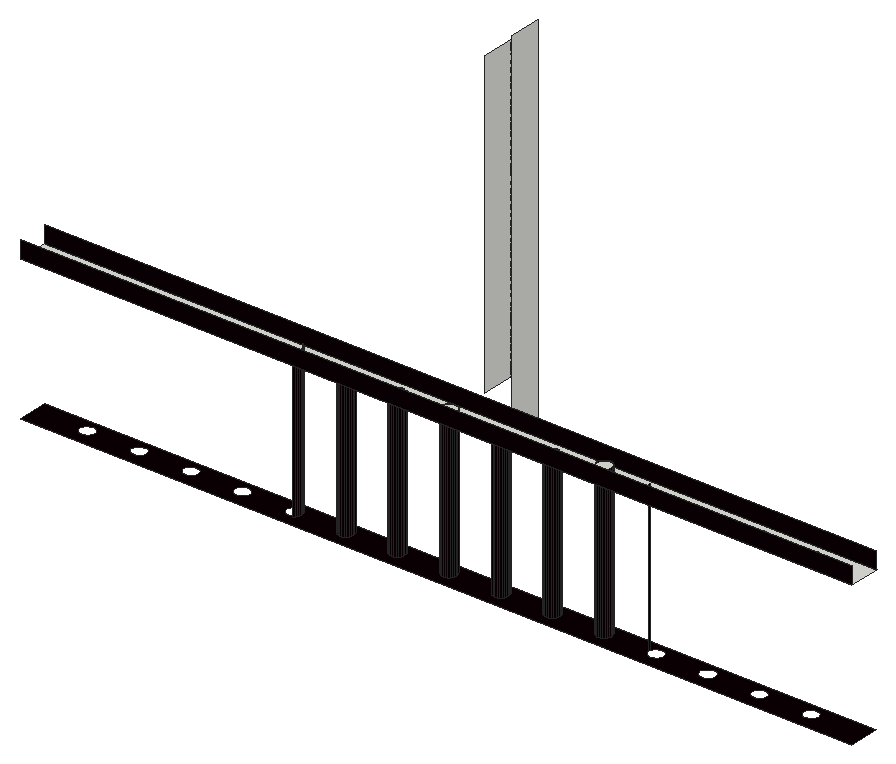
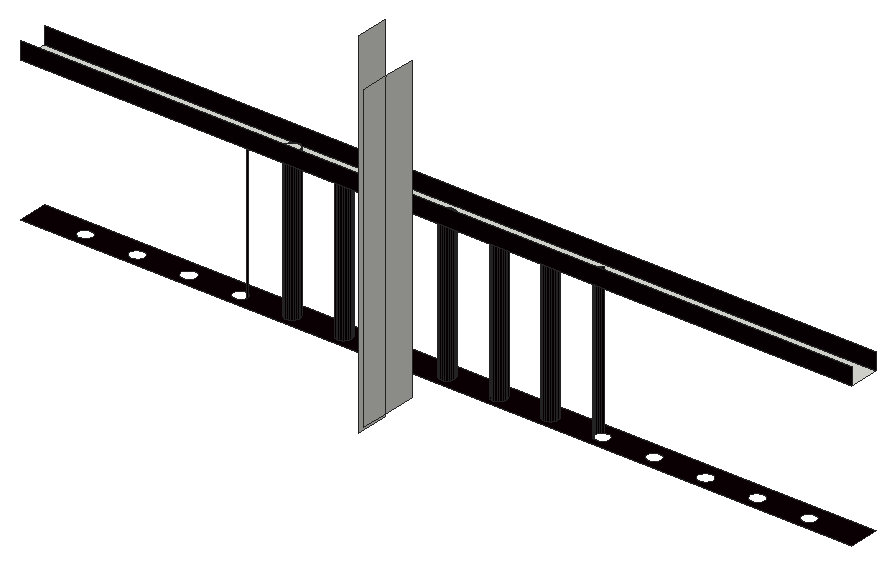
# SketchUp Ruby script. Lengths in inches.
U = 1.inch
M = Sketchup.active_model
def pt(a) = Geom::Point3d.new(a.map { |v| v * U })
def face(e, loops, mat)
  f = e.add_face(loops[0].map { |a| pt(a) })
  loops[1..].each { |l| e.add_face(l.map { |a| pt(a) }).erase! }
  f.material = f.back_material = mat if mat
  f
end
# faces: each face lists its corners as indices into pts; further lists are holes
def faces(e, pts, list, mat = nil) = list.each { |f| face(e, (f[0].is_a?(Array) ? f : [f]).map { |l| l.map { |i| pts[i] } }, mat) }
# xy, xz, yz: faces in a plane at the given z, y or x. An outline is a flat list of corners, or four numbers for a rectangle; further outlines are holes
def ring(l) = l.size == 4 ? [[l[0], l[1]], [l[2], l[1]], [l[2], l[3]], [l[0], l[3]]] : l.each_slice(2).to_a
def flat(e, list, mat, &to3) = list.each { |f| face(e, (f[0].is_a?(Array) ? f : [f]).map { |l| ring(l).map { |u, v| to3.(u, v) } }, mat) }
def xy(e, z, list, mat = nil) = flat(e, list, mat) { |x, y| [x, y, z] }
def xz(e, y, list, mat = nil) = flat(e, list, mat) { |x, z| [x, y, z] }
def yz(e, x, list, mat = nil) = flat(e, list, mat) { |y, z| [x, y, z] }
def lines(e, pts, list) = list.each { |a, b| e.add_line(pt(pts[a]), pt(pts[b])) }
# prism: a flat outline (further loops are holes) pulled along v
def prism(e, loops, v, mat = nil)
  f = face(e, loops, mat); d = Geom::Vector3d.new(v.map { |x| x * U })
  f.pushpull(f.normal.samedirection?(d) ? d.length : -d.length)
end
def box(e, o, s, mat = nil) = prism(e, [[o, [o[0] + s[0], o[1], o[2]], [o[0] + s[0], o[1] + s[1], o[2]], [o[0], o[1] + s[1], o[2]]]], [0, 0, s[2]], mat)
def at(x, y, z, deg = 0) = Geom::Transformation.translation(pt([x, y, z])) * Geom::Transformation.rotation(ORIGIN, Z_AXIS, deg.degrees)
def axes(o, x, y, z) = Geom::Transformation.new([*x, 0, *y, 0, *z, 0, *pt(o).to_a, 1])
def part(name) = M.definitions.add(name)
# library, detail: a bought-in or finely detailed component or shape, given as its bounding box
def library(name, o, s) = part(name).tap { |d| box(d.entities, o, s) }
def detail(e, o, s) = box(e.add_group.entities, o, s)
def put(e, d, t, mat = nil) = e.add_instance(d, t).tap { |i| i.material = mat if mat }
def group(e, t, mat = nil) = e.add_group.tap { |g| g.transformation = t; g.material = mat if mat }.entities
root = M.entities
M.materials.add("[Metal Seamed]").color = [11, 0, 4]
xy(root,156,[[439.47,72.62,439.03,72.67,438.62,72.83,438.26,73.09,437.99,73.43,437.8125,73.83,437.75,74.27,437.79,74.71,437.95,75.12,438.21,75.47,438.56,75.75,438.96,75.93,439.4,75.99,439.83,75.94,440.25,75.78,440.6,75.52,440.875,75.18,441.05,74.78,441.12,74.34,441.07,73.9,440.91,73.49,440.65,73.14,440.31,72.86,439.9,72.68],[451.09,72.62,450.66,72.67,450.25,72.83,449.89,73.09,449.61,73.43,449.4375,73.83,449.37,74.27,449.42,74.71,449.58,75.12,449.84,75.47,450.18,75.75,450.59,75.93,451.02,75.99,451.46,75.94,451.87,75.78,452.23,75.52,452.5,75.18,452.68,74.78,452.74,74.34,452.7,73.9,452.54,73.49,452.28,73.14,451.93,72.86,451.53,72.68],[462.72,72.62,462.28,72.67,461.87,72.83,461.51,73.09,461.24,73.43,461.0625,73.83,461,74.27,461.04,74.71,461.2,75.12,461.46,75.47,461.81,75.75,462.21,75.93,462.65,75.99,463.08,75.94,463.5,75.78,463.85,75.52,464.125,75.18,464.3,74.78,464.37,74.34,464.32,73.9,464.16,73.49,463.9,73.14,463.56,72.86,463.15,72.68],[474.34,72.62,473.91,72.67,473.5,72.83,473.14,73.09,472.86,73.43,472.6875,73.83,472.62,74.27,472.67,74.71,472.83,75.12,473.09,75.47,473.43,75.75,473.84,75.93,474.27,75.99,474.71,75.94,475.12,75.78,475.48,75.52,475.75,75.18,475.93,74.78,475.99,74.34,475.95,73.9,475.79,73.49,475.53,73.14,475.18,72.86,474.78,72.68],[485.97,72.62,485.53,72.67,485.12,72.83,484.76,73.09,484.49,73.43,484.3125,73.83,484.25,74.27,484.29,74.71,484.45,75.12,484.71,75.47,485.06,75.75,485.46,75.93,485.9,75.99,486.33,75.94,486.75,75.78,487.1,75.52,487.375,75.18,487.55,74.78,487.62,74.34,487.57,73.9,487.41,73.49,487.15,73.14,486.81,72.86,486.4,72.68],
  [497.59,72.62,497.16,72.67,496.75,72.83,496.39,73.09,496.11,73.43,495.9375,73.83,495.87,74.27,495.92,74.71,496.08,75.12,496.34,75.47,496.68,75.75,497.09,75.93,497.52,75.99,497.96,75.94,498.37,75.78,498.73,75.52,499,75.18,499.18,74.78,499.24,74.34,499.2,73.9,499.04,73.49,498.78,73.14,498.43,72.86,498.03,72.68]])
xy(root,156,[[[369.3125,70.41,556.3,77.3],[381.34,72.62,380.91,72.67,380.5,72.83,380.14,73.09,379.86,73.43,379.6875,73.83,379.62,74.27,379.67,74.71,379.83,75.12,380.09,75.47,380.43,75.75,380.84,75.93,381.27,75.99,381.71,75.94,382.12,75.78,382.48,75.52,382.75,75.18,382.93,74.78,382.99,74.34,382.95,73.9,382.79,73.49,382.53,73.14,382.18,72.86,381.78,72.68],[392.97,72.62,392.53,72.67,392.12,72.83,391.76,73.09,391.49,73.43,391.3125,73.83,391.25,74.27,391.29,74.71,391.45,75.12,391.71,75.47,392.06,75.75,392.46,75.93,392.9,75.99,393.33,75.94,393.75,75.78,394.1,75.52,394.375,75.18,394.55,74.78,394.62,74.34,394.57,73.9,394.41,73.49,394.15,73.14,393.81,72.86,393.4,72.68],[404.59,72.62,404.16,72.67,403.75,72.83,403.39,73.09,403.11,73.43,402.9375,73.83,402.87,74.27,402.92,74.71,403.08,75.12,403.34,75.47,403.68,75.75,404.09,75.93,404.52,75.99,404.96,75.94,405.37,75.78,405.73,75.52,406,75.18,406.18,74.78,406.24,74.34,406.2,73.9,406.04,73.49,405.78,73.14,405.43,72.86,405.03,72.68],[416.22,72.62,415.78,72.67,415.37,72.83,415.01,73.09,414.74,73.43,414.5625,73.83,414.5,74.27,414.54,74.71,414.7,75.12,414.96,75.47,415.31,75.75,415.71,75.93,416.15,75.99,416.58,75.94,417,75.78,417.35,75.52,417.625,75.18,417.8,74.78,417.87,74.34,417.82,73.9,417.66,73.49,417.4,73.14,417.06,72.86,416.65,72.68],[427.84,72.62,427.41,72.67,427,72.83,426.64,73.09,426.36,73.43,426.1875,73.83,426.12,74.27,426.17,74.71,426.33,75.12,426.59,75.47,426.93,75.75,427.34,75.93,427.77,75.99,428.21,75.94,428.62,75.78,428.98,75.52,429.25,75.18,429.43,74.78,429.49,74.34,429.45,73.9,429.29,73.49,429.03,73.14,428.68,72.86,428.28,72.68],[439.47,72.62,439.03,72.67,438.62,72.83,438.26,73.09,437.99,73.43,437.8125,73.83,437.75,74.27,437.79,74.71,437.95,75.12,438.21,75.47,438.56,75.75,438.96,75.93,439.4,75.99,439.83,75.94,440.25,75.78,440.6,75.52,440.875,75.18,441.05,74.78,441.12,74.34,441.07,73.9,440.91,73.49,440.65,73.14,440.31,72.86,439.9,72.68],[451.09,72.62,450.66,72.67,450.25,72.83,449.89,73.09,449.61,73.43,449.4375,73.83,449.37,74.27,449.42,74.71,449.58,75.12,449.84,75.47,450.18,75.75,450.59,75.93,451.02,75.99,451.46,75.94,451.87,75.78,452.23,75.52,452.5,75.18,452.68,74.78,452.74,74.34,452.7,73.9,452.54,73.49,452.28,73.14,451.93,72.86,451.53,72.68],[462.72,72.62,462.28,72.67,461.87,72.83,461.51,73.09,461.24,73.43,461.0625,73.83,461,74.27,461.04,74.71,461.2,75.12,461.46,75.47,461.81,75.75,462.21,75.93,462.65,75.99,463.08,75.94,463.5,75.78,463.85,75.52,464.125,75.18,464.3,74.78,464.37,74.34,464.32,73.9,464.16,73.49,463.9,73.14,463.56,72.86,463.15,72.68],[474.34,72.62,473.91,72.67,473.5,72.83,473.14,73.09,472.86,73.43,472.6875,73.83,472.62,74.27,472.67,74.71,472.83,75.12,473.09,75.47,473.43,75.75,473.84,75.93,474.27,75.99,474.71,75.94,475.12,75.78,475.48,75.52,475.75,75.18,475.93,74.78,475.99,74.34,475.95,73.9,475.79,73.49,475.53,73.14,475.18,72.86,474.78,72.68],[485.97,72.62,485.53,72.67,485.12,72.83,484.76,73.09,484.49,73.43,484.3125,73.83,484.25,74.27,484.29,74.71,484.45,75.12,484.71,75.47,485.06,75.75,485.46,75.93,485.9,75.99,486.33,75.94,486.75,75.78,487.1,75.52,487.375,75.18,487.55,74.78,487.62,74.34,487.57,73.9,487.41,73.49,487.15,73.14,486.81,72.86,486.4,72.68],[497.59,72.62,497.16,72.67,496.75,72.83,496.39,73.09,496.11,73.43,495.9375,73.83,495.87,74.27,495.92,74.71,496.08,75.12,496.34,75.47,496.68,75.75,497.09,75.93,497.52,75.99,497.96,75.94,498.37,75.78,498.73,75.52,499,75.18,499.18,74.78,499.24,74.34,499.2,73.9,499.04,73.49,498.78,73.14,498.43,72.86,498.03,72.68],[509.22,72.62,508.78,72.67,508.37,72.83,508.01,73.09,507.74,73.43,507.5625,73.83,507.5,74.27,507.54,74.71,507.7,75.12,507.96,75.47,508.31,75.75,508.71,75.93,509.15,75.99,509.58,75.94,510,75.78,510.35,75.52,510.625,75.18,510.8,74.78,510.87,74.34,510.82,73.9,510.66,73.49,510.4,73.14,510.06,72.86,509.65,72.68],[520.84,72.62,520.41,72.67,520,72.83,519.64,73.09,519.36,73.43,519.1875,73.83,519.12,74.27,519.17,74.71,519.33,75.12,519.59,75.47,519.93,75.75,520.34,75.93,520.77,75.99,521.21,75.94,521.62,75.78,521.98,75.52,522.25,75.18,522.43,74.78,522.49,74.34,522.45,73.9,522.29,73.49,522.03,73.14,521.68,72.86,521.28,72.68],[532.47,72.62,532.03,72.67,531.62,72.83,531.26,73.09,530.99,73.43,530.8125,73.83,530.75,74.27,530.79,74.71,530.95,75.12,531.21,75.47,531.56,75.75,531.96,75.93,532.4,75.99,532.83,75.94,533.25,75.78,533.6,75.52,533.875,75.18,534.05,74.78,534.12,74.34,534.07,73.9,533.91,73.49,533.65,73.14,533.31,72.86,532.9,72.68],[544.09,72.62,543.66,72.67,543.25,72.83,542.89,73.09,542.61,73.43,542.4375,73.83,542.37,74.27,542.42,74.71,542.58,75.12,542.84,75.47,543.18,75.75,543.59,75.93,544.02,75.99,544.46,75.94,544.87,75.78,545.23,75.52,545.5,75.18,545.68,74.78,545.74,74.34,545.7,73.9,545.54,73.49,545.28,73.14,544.93,72.86,544.53,72.68]]],"[Metal Seamed]")
xy(root,187.8125,[[439.47,72.62,439.9,72.68,440.31,72.86,440.65,73.14,440.91,73.49,441.07,73.9,441.12,74.34,441.05,74.78,440.875,75.18,440.6,75.52,440.25,75.78,439.83,75.94,439.4,75.99,438.96,75.93,438.56,75.75,438.21,75.47,437.95,75.12,437.79,74.71,437.75,74.27,437.8125,73.83,437.99,73.43,438.26,73.09,438.62,72.83,439.03,72.67],[474.34,72.62,474.78,72.68,475.18,72.86,475.53,73.14,475.79,73.49,475.95,73.9,475.99,74.34,475.93,74.78,475.75,75.18,475.48,75.52,475.12,75.78,474.71,75.94,474.27,75.99,473.84,75.93,473.43,75.75,473.09,75.47,472.83,75.12,472.67,74.71,472.62,74.27,472.6875,73.83,472.86,73.43,473.14,73.09,473.5,72.83,473.91,72.67]])
xy(root,188.2,[[[369.3125,70.41,556.3125,77.3],[392.97,72.62,393.4,72.68,393.81,72.86,394.15,73.14,394.41,73.49,394.57,73.9,394.62,74.34,394.55,74.78,394.375,75.18,394.1,75.52,393.75,75.78,393.33,75.94,392.9,75.99,392.46,75.93,392.06,75.75,391.71,75.47,391.45,75.12,391.29,74.71,391.25,74.27,391.3125,73.83,391.49,73.43,391.76,73.09,392.12,72.83,392.53,72.67],[451.09,72.62,451.53,72.68,451.93,72.86,452.28,73.14,452.54,73.49,452.7,73.9,452.74,74.34,452.68,74.78,452.5,75.18,452.23,75.52,451.87,75.78,451.46,75.94,451.02,75.99,450.59,75.93,450.18,75.75,449.84,75.47,449.58,75.12,449.42,74.71,449.37,74.27,449.4375,73.83,449.61,73.43,449.89,73.09,450.25,72.83,450.66,72.67],[485.97,72.62,486.4,72.68,486.81,72.86,487.15,73.14,487.41,73.49,487.57,73.9,487.62,74.34,487.55,74.78,487.375,75.18,487.1,75.52,486.75,75.78,486.33,75.94,485.9,75.99,485.46,75.93,485.06,75.75,484.71,75.47,484.45,75.12,484.29,74.71,484.25,74.27,484.3125,73.83,484.49,73.43,484.76,73.09,485.12,72.83,485.53,72.67],[532.47,72.62,532.9,72.68,533.31,72.86,533.65,73.14,533.91,73.49,534.07,73.9,534.12,74.34,534.05,74.78,533.875,75.18,533.6,75.52,533.25,75.78,532.83,75.94,532.4,75.99,531.96,75.93,531.56,75.75,531.21,75.47,530.95,75.12,530.79,74.71,530.75,74.27,530.8125,73.83,530.99,73.43,531.26,73.09,531.62,72.83,532.03,72.67],[544.09,72.62,544.53,72.68,544.93,72.86,545.28,73.14,545.54,73.49,545.7,73.9,545.74,74.34,545.68,74.78,545.5,75.18,545.23,75.52,544.87,75.78,544.46,75.94,544.02,75.99,543.59,75.93,543.18,75.75,542.84,75.47,542.58,75.12,542.42,74.71,542.37,74.27,542.4375,73.83,542.61,73.43,542.89,73.09,543.25,72.83,543.66,72.67]]])
xy(root,189.0625,[[462.72,72.62,463.15,72.68,463.56,72.86,463.9,73.14,464.16,73.49,464.32,73.9,464.37,74.34,464.3,74.78,464.125,75.18,463.85,75.52,463.5,75.78,463.08,75.94,462.65,75.99,462.21,75.93,461.81,75.75,461.46,75.47,461.2,75.12,461.04,74.71,461,74.27,461.0625,73.83,461.24,73.43,461.51,73.09,461.87,72.83,462.28,72.67]])
xy(root,189.9375,[[497.59,72.62,498.03,72.68,498.43,72.86,498.78,73.14,499.04,73.49,499.2,73.9,499.24,74.34,499.18,74.78,499,75.18,498.73,75.52,498.37,75.78,497.96,75.94,497.52,75.99,497.09,75.93,496.68,75.75,496.34,75.47,496.08,75.12,495.92,74.71,495.87,74.27,495.9375,73.83,496.11,73.43,496.39,73.09,496.75,72.83,497.16,72.67]])
xz(root,70.41,[[369.3125,188.2,556.3,192]],"[Metal Seamed]")
xz(root,77.3,[[369.3125,188.2,556.3,192]],"[Metal Seamed]")
yz(root,445.08,[[106.41,171.98,113.66,239.92],[113.66,171.98,119.66,239.92]])
yz(root,451.12,[[106.41,165.94,113.66,245.96]])
p = [[439.03,72.67,156],[439.47,72.62,156],[439.47,72.62,187.8125],[439.03,72.67,187.8125],[439.9,72.68,156],[439.9,72.68,187.8125],
  [450.66,72.67,156],[451.09,72.62,156],[451.09,72.62,188.2],[450.66,72.67,188.2],[451.53,72.68,156],[451.53,72.68,188.2],
  [462.28,72.67,156],[462.72,72.62,156],[462.72,72.62,189.0625],[462.28,72.67,189.0625],[463.15,72.68,156],[463.15,72.68,189.0625],
  [473.91,72.67,156],[474.34,72.62,156],[474.34,72.62,187.8125],[473.91,72.67,187.8125],[474.78,72.68,156],[474.78,72.68,187.8125],
  [485.53,72.67,156],[485.97,72.62,156],[485.97,72.62,188.2],[485.53,72.67,188.2],[486.4,72.68,156],[486.4,72.68,188.2],
  [497.16,72.67,156],[497.59,72.62,156],[497.59,72.62,189.9375],[497.16,72.67,189.9375],[498.03,72.68,156],[498.03,72.68,189.9375],
  [438.62,72.83,156],[438.62,72.83,187.8125],[440.31,72.86,156],[440.31,72.86,187.8125],[450.25,72.83,156],[450.25,72.83,188.2],
  [451.93,72.86,156],[451.93,72.86,188.2],[461.87,72.83,156],[461.87,72.83,189.0625],[463.56,72.86,156],[463.56,72.86,189.0625],
  [473.5,72.83,156],[473.5,72.83,187.8125],[475.18,72.86,156],[475.18,72.86,187.8125],[485.12,72.83,156],[485.12,72.83,188.2],
  [486.81,72.86,156],[486.81,72.86,188.2],[496.75,72.83,156],[496.75,72.83,189.9375],[498.43,72.86,156],[498.43,72.86,189.9375],
  [438.26,73.09,156],[438.26,73.09,187.8125],[449.89,73.09,156],[449.89,73.09,188.2],[461.51,73.09,156],[461.51,73.09,189.0625],
  [473.14,73.09,156],[473.14,73.09,187.8125],[484.76,73.09,156],[484.76,73.09,188.2],[496.39,73.09,156],[496.39,73.09,189.9375],
  [428.68,72.86,156],[429.03,73.14,156],[429.03,73.14,189.4375],[428.68,72.86,189.4375],[440.65,73.14,156],[440.65,73.14,187.8125],
  [452.28,73.14,156],[452.28,73.14,188.2],[463.9,73.14,156],[463.9,73.14,189.0625],[475.53,73.14,156],[475.53,73.14,187.8125],
  [487.15,73.14,156],[487.15,73.14,188.2],[498.78,73.14,156],[498.78,73.14,189.9375],[429.29,73.49,156],[429.29,73.49,189.4375],
  [437.99,73.43,156],[437.99,73.43,187.8125],[440.91,73.49,156],[440.91,73.49,187.8125],[449.61,73.43,156],[449.61,73.43,188.2],
  [452.54,73.49,156],[452.54,73.49,188.2],[461.24,73.43,156],[461.24,73.43,189.0625],[464.16,73.49,156],[464.16,73.49,189.0625],
  [472.86,73.43,156],[472.86,73.43,187.8125],[475.79,73.49,156],[475.79,73.49,187.8125],[484.49,73.43,156],[484.49,73.43,188.2],
  [487.41,73.49,156],[487.41,73.49,188.2],[496.11,73.43,156],[496.11,73.43,189.9375],[499.04,73.49,156],[499.04,73.49,189.9375],
  [437.8125,73.83,156],[437.8125,73.83,187.8125],[449.4375,73.83,156],[449.4375,73.83,188.2],[461.0625,73.83,156],[461.0625,73.83,189.0625],
  [472.6875,73.83,156],[472.6875,73.83,187.8125],[484.3125,73.83,156],[484.3125,73.83,188.2],[495.9375,73.83,156],[495.9375,73.83,189.9375],
  [429.45,73.9,156],[429.45,73.9,189.4375],[441.07,73.9,156],[441.07,73.9,187.8125],[452.7,73.9,156],[452.7,73.9,188.2],
  [464.32,73.9,156],[464.32,73.9,189.0625],[475.95,73.9,156],[475.95,73.9,187.8125],[487.57,73.9,156],[487.57,73.9,188.2],
  [499.2,73.9,156],[499.2,73.9,189.9375],[437.75,74.27,156],[437.75,74.27,187.8125],[449.37,74.27,156],[449.37,74.27,188.2],
  [461,74.27,156],[461,74.27,189.0625],[472.62,74.27,156],[472.62,74.27,187.8125],[484.25,74.27,156],[484.25,74.27,188.2],
  [495.87,74.27,156],[495.87,74.27,189.9375],[429.49,74.34,156],[429.49,74.34,189.4375],[441.12,74.34,156],[441.12,74.34,187.8125],
  [452.74,74.34,156],[452.74,74.34,188.2],[464.37,74.34,156],[464.37,74.34,189.0625],[475.99,74.34,156],[475.99,74.34,187.8125],
  [487.62,74.34,156],[487.62,74.34,188.2],[499.24,74.34,156],[499.24,74.34,189.9375],[429.43,74.78,156],[429.43,74.78,189.4375],
  [437.79,74.71,156],[437.79,74.71,187.8125],[441.05,74.78,156],[441.05,74.78,187.8125],[449.42,74.71,156],[449.42,74.71,188.2],
  [452.68,74.78,156],[452.68,74.78,188.2],[461.04,74.71,156],[461.04,74.71,189.0625],[464.3,74.78,156],[464.3,74.78,189.0625],
  [472.67,74.71,156],[472.67,74.71,187.8125],[475.93,74.78,156],[475.93,74.78,187.8125],[484.29,74.71,156],[484.29,74.71,188.2],
  [487.55,74.78,156],[487.55,74.78,188.2],[495.92,74.71,156],[495.92,74.71,189.9375],[499.18,74.78,156],[499.18,74.78,189.9375],
  [507.54,74.71,156],[507.5,74.27,156],[507.5,74.27,189.4375],[507.54,74.71,189.4375],[437.95,75.12,156],[437.95,75.12,187.8125],
  [449.58,75.12,156],[449.58,75.12,188.2],[461.2,75.12,156],[461.2,75.12,189.0625],[472.83,75.12,156],[472.83,75.12,187.8125],
  [484.45,75.12,156],[484.45,75.12,188.2],[496.08,75.12,156],[496.08,75.12,189.9375],[429.25,75.18,156],[429.25,75.18,189.4375],
  [440.875,75.18,156],[440.875,75.18,187.8125],[452.5,75.18,156],[452.5,75.18,188.2],[464.125,75.18,156],[464.125,75.18,189.0625],
  [475.75,75.18,156],[475.75,75.18,187.8125],[487.375,75.18,156],[487.375,75.18,188.2],[499,75.18,156],[499,75.18,189.9375],
  [438.21,75.47,156],[438.21,75.47,187.8125],[449.84,75.47,156],[449.84,75.47,188.2],[461.46,75.47,156],[461.46,75.47,189.0625],
  [473.09,75.47,156],[473.09,75.47,187.8125],[484.71,75.47,156],[484.71,75.47,188.2],[496.34,75.47,156],[496.34,75.47,189.9375],
  [428.98,75.52,156],[428.98,75.52,189.4375],[440.6,75.52,156],[440.6,75.52,187.8125],[452.23,75.52,156],[452.23,75.52,188.2],
  [463.85,75.52,156],[463.85,75.52,189.0625],[475.48,75.52,156],[475.48,75.52,187.8125],[487.1,75.52,156],[487.1,75.52,188.2],
  [498.73,75.52,156],[498.73,75.52,189.9375],[428.62,75.78,156],[428.62,75.78,189.4375],[438.56,75.75,156],[438.56,75.75,187.8125],
  [440.25,75.78,156],[440.25,75.78,187.8125],[450.18,75.75,156],[450.18,75.75,188.2],[451.87,75.78,156],[451.87,75.78,188.2],
  [461.81,75.75,156],[461.81,75.75,189.0625],[463.5,75.78,156],[463.5,75.78,189.0625],[473.43,75.75,156],[473.43,75.75,187.8125],
  [475.12,75.78,156],[475.12,75.78,187.8125],[485.06,75.75,156],[485.06,75.75,188.2],[486.75,75.78,156],[486.75,75.78,188.2],
  [496.68,75.75,156],[496.68,75.75,189.9375],[498.37,75.78,156],[498.37,75.78,189.9375],[438.96,75.93,156],[438.96,75.93,187.8125],
  [450.59,75.93,156],[450.59,75.93,188.2],[462.21,75.93,156],[462.21,75.93,189.0625],[473.84,75.93,156],[473.84,75.93,187.8125],
  [485.46,75.93,156],[485.46,75.93,188.2],[497.09,75.93,156],[497.09,75.93,189.9375],[439.83,75.94,156],[439.83,75.94,187.8125],
  [451.46,75.94,156],[451.46,75.94,188.2],[463.08,75.94,156],[463.08,75.94,189.0625],[474.71,75.94,156],[474.71,75.94,187.8125],
  [486.33,75.94,156],[486.33,75.94,188.2],[497.96,75.94,156],[497.96,75.94,189.9375],[439.4,75.99,156],[439.4,75.99,187.8125],
  [451.02,75.99,156],[451.02,75.99,188.2],[462.65,75.99,156],[462.65,75.99,189.0625],[474.27,75.99,156],[474.27,75.99,187.8125],
  [485.9,75.99,156],[485.9,75.99,188.2],[497.52,75.99,156],[497.52,75.99,189.9375]]
faces(root,p,[[0,1,2,3],[1,4,5,2],[6,7,8,9],[7,10,11,8],[12,13,14,15],[13,16,17,14],[18,19,20,21],[19,22,23,20],
  [24,25,26,27],[25,28,29,26],[30,31,32,33],[31,34,35,32],[36,0,3,37],[4,38,39,5],[40,6,9,41],[10,42,43,11],
  [44,12,15,45],[16,46,47,17],[48,18,21,49],[22,50,51,23],[52,24,27,53],[28,54,55,29],[56,30,33,57],[34,58,59,35],
  [60,36,37,61],[62,40,41,63],[64,44,45,65],[66,48,49,67],[68,52,53,69],[70,56,57,71],[72,73,74,75],[38,76,77,39],
  [42,78,79,43],[46,80,81,47],[50,82,83,51],[54,84,85,55],[58,86,87,59],[73,88,89,74],[90,60,61,91],[76,92,93,77],
  [94,62,63,95],[78,96,97,79],[98,64,65,99],[80,100,101,81],[102,66,67,103],[82,104,105,83],[106,68,69,107],[84,108,109,85],
  [110,70,71,111],[86,112,113,87],[114,90,91,115],[116,94,95,117],[118,98,99,119],[120,102,103,121],[122,106,107,123],[124,110,111,125],
  [88,126,127,89],[92,128,129,93],[96,130,131,97],[100,132,133,101],[104,134,135,105],[108,136,137,109],[112,138,139,113],[140,114,115,141],
  [142,116,117,143],[144,118,119,145],[146,120,121,147],[148,122,123,149],[150,124,125,151],[126,152,153,127],[128,154,155,129],[130,156,157,131],
  [132,158,159,133],[134,160,161,135],[136,162,163,137],[138,164,165,139],[152,166,167,153],[168,140,141,169],[154,170,171,155],[172,142,143,173],
  [156,174,175,157],[176,144,145,177],[158,178,179,159],[180,146,147,181],[160,182,183,161],[184,148,149,185],[162,186,187,163],[188,150,151,189],
  [164,190,191,165],[192,193,194,195],[196,168,169,197],[198,172,173,199],[200,176,177,201],[202,180,181,203],[204,184,185,205],[206,188,189,207],
  [166,208,209,167],[170,210,211,171],[174,212,213,175],[178,214,215,179],[182,216,217,183],[186,218,219,187],[190,220,221,191],[222,196,197,223],
  [224,198,199,225],[226,200,201,227],[228,202,203,229],[230,204,205,231],[232,206,207,233],[208,234,235,209],[210,236,237,211],[212,238,239,213],
  [214,240,241,215],[216,242,243,217],[218,244,245,219],[220,246,247,221],[234,248,249,235],[250,222,223,251],[236,252,253,237],[254,224,225,255],
  [238,256,257,239],[258,226,227,259],[240,260,261,241],[262,228,229,263],[242,264,265,243],[266,230,231,267],[244,268,269,245],[270,232,233,271],
  [246,272,273,247],[274,250,251,275],[276,254,255,277],[278,258,259,279],[280,262,263,281],[282,266,267,283],[284,270,271,285],[252,286,287,253],
  [256,288,289,257],[260,290,291,261],[264,292,293,265],[268,294,295,269],[272,296,297,273],[298,274,275,299],[286,298,299,287],[300,276,277,301],
  [288,300,301,289],[302,278,279,303],[290,302,303,291],[304,280,281,305],[292,304,305,293],[306,282,283,307],[294,306,307,295],[308,284,285,309],
  [296,308,309,297]],"[Metal Seamed]")
